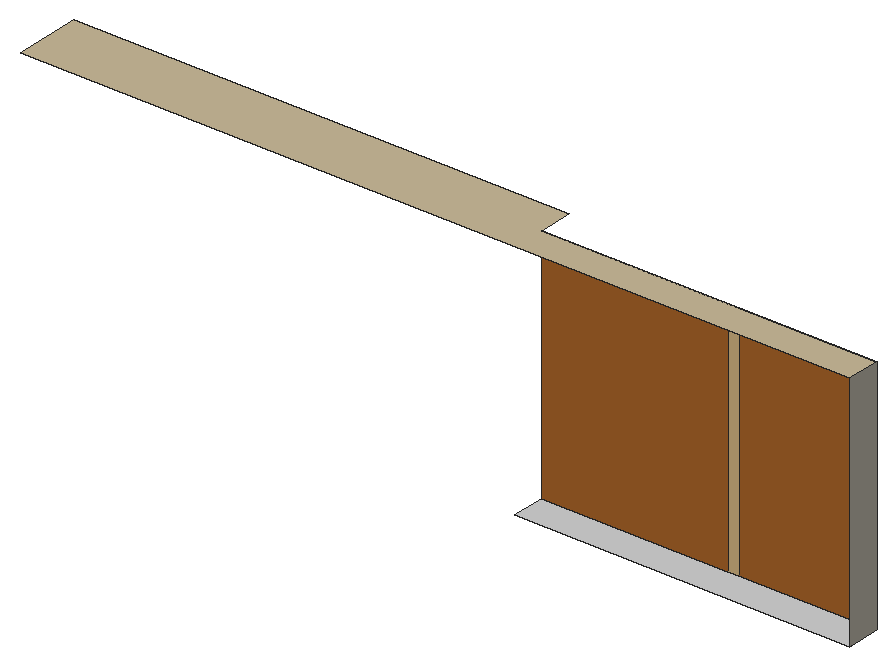
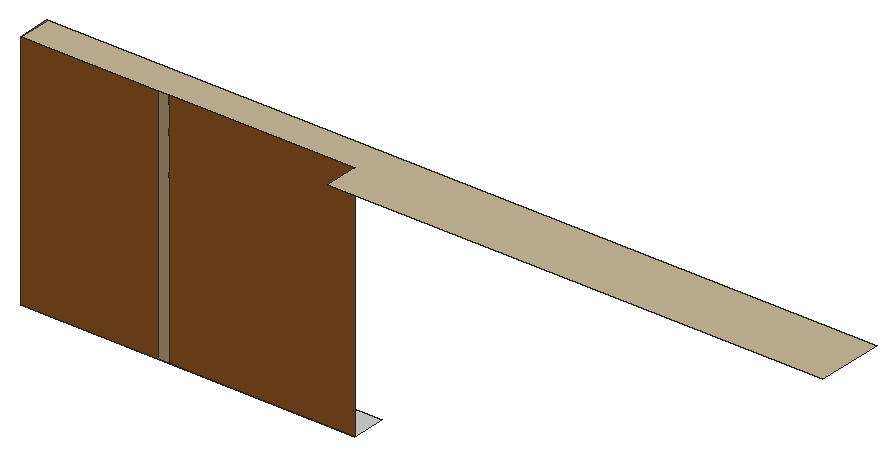
# SketchUp Ruby script. Lengths in inches.
U = 1.inch
M = Sketchup.active_model
def pt(a) = Geom::Point3d.new(a.map { |v| v * U })
def face(e, loops, mat)
  f = e.add_face(loops[0].map { |a| pt(a) })
  loops[1..].each { |l| e.add_face(l.map { |a| pt(a) }).erase! }
  f.material = f.back_material = mat if mat
  f
end
# faces: each face lists its corners as indices into pts; further lists are holes
def faces(e, pts, list, mat = nil) = list.each { |f| face(e, (f[0].is_a?(Array) ? f : [f]).map { |l| l.map { |i| pts[i] } }, mat) }
# xy, xz, yz: faces in a plane at the given z, y or x. An outline is a flat list of corners, or four numbers for a rectangle; further outlines are holes
def ring(l) = l.size == 4 ? [[l[0], l[1]], [l[2], l[1]], [l[2], l[3]], [l[0], l[3]]] : l.each_slice(2).to_a
def flat(e, list, mat, &to3) = list.each { |f| face(e, (f[0].is_a?(Array) ? f : [f]).map { |l| ring(l).map { |u, v| to3.(u, v) } }, mat) }
def xy(e, z, list, mat = nil) = flat(e, list, mat) { |x, y| [x, y, z] }
def xz(e, y, list, mat = nil) = flat(e, list, mat) { |x, z| [x, y, z] }
def yz(e, x, list, mat = nil) = flat(e, list, mat) { |y, z| [x, y, z] }
def lines(e, pts, list) = list.each { |a, b| e.add_line(pt(pts[a]), pt(pts[b])) }
# prism: a flat outline (further loops are holes) pulled along v
def prism(e, loops, v, mat = nil)
  f = face(e, loops, mat); d = Geom::Vector3d.new(v.map { |x| x * U })
  f.pushpull(f.normal.samedirection?(d) ? d.length : -d.length)
end
def box(e, o, s, mat = nil) = prism(e, [[o, [o[0] + s[0], o[1], o[2]], [o[0] + s[0], o[1] + s[1], o[2]], [o[0], o[1] + s[1], o[2]]]], [0, 0, s[2]], mat)
def at(x, y, z, deg = 0) = Geom::Transformation.translation(pt([x, y, z])) * Geom::Transformation.rotation(ORIGIN, Z_AXIS, deg.degrees)
def axes(o, x, y, z) = Geom::Transformation.new([*x, 0, *y, 0, *z, 0, *pt(o).to_a, 1])
def part(name) = M.definitions.add(name)
# library, detail: a bought-in or finely detailed component or shape, given as its bounding box
def library(name, o, s) = part(name).tap { |d| box(d.entities, o, s) }
def detail(e, o, s) = box(e.add_group.entities, o, s)
def put(e, d, t, mat = nil) = e.add_instance(d, t).tap { |i| i.material = mat if mat }
def group(e, t, mat = nil) = e.add_group.tap { |g| g.transformation = t; g.material = mat if mat }.entities
root = M.entities
M.materials.add("[Carrera Marble]").color = [207, 207, 207]
M.materials.add("[Formica Graystone]").color = [149, 146, 135]
M.materials.add("[Quartz Light Brown]").color = [199, 184, 152]
M.materials.add("[Wood Bamboo]").color = [165, 98, 40]
M.materials.add("[Wood Floor Light]").color = [204, 176, 127]
xy(root,0,[[201.37,184.11,321.5,196.19]],"[Carrera Marble]")
xy(root,86.16,[[24.17,184.11,24.17,208.28,201.37,208.28,201.37,196.19,321.5,196.19,321.5,184.11]],"[Quartz Light Brown]")
xz(root,196.19,[[201.37,0,268.28,86.16],[272.19,0,321.5,86.16]],"[Wood Bamboo]")
xz(root,196.19,[[268.28,0,272.19,86.16]],"[Wood Floor Light]")
yz(root,321.5,[[184.11,0,196.19,86.16]],"[Formica Graystone]")
